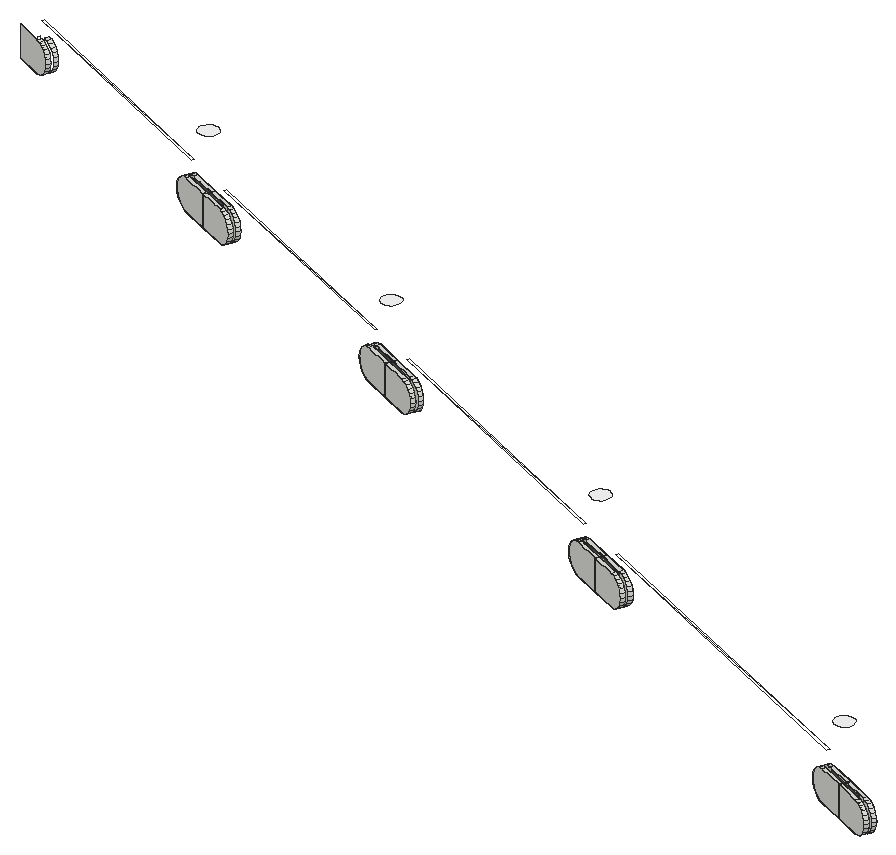
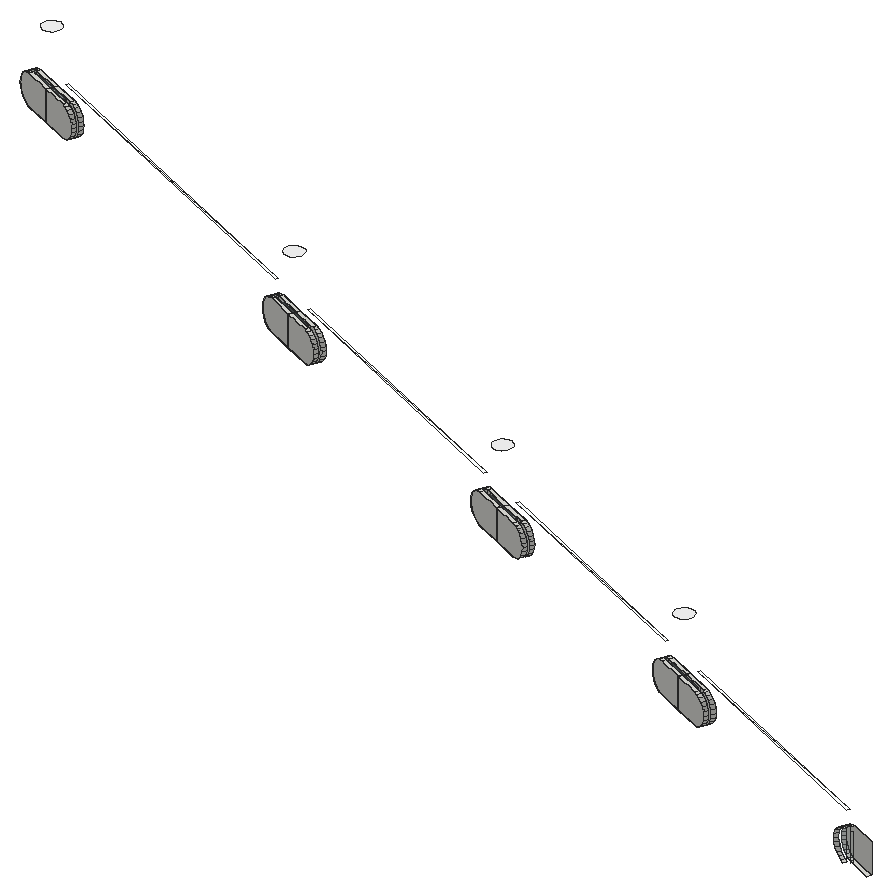
# SketchUp Ruby script. Lengths in inches.
U = 1.inch
M = Sketchup.active_model
def pt(a) = Geom::Point3d.new(a.map { |v| v * U })
def face(e, loops, mat)
  f = e.add_face(loops[0].map { |a| pt(a) })
  loops[1..].each { |l| e.add_face(l.map { |a| pt(a) }).erase! }
  f.material = f.back_material = mat if mat
  f
end
# faces: each face lists its corners as indices into pts; further lists are holes
def faces(e, pts, list, mat = nil) = list.each { |f| face(e, (f[0].is_a?(Array) ? f : [f]).map { |l| l.map { |i| pts[i] } }, mat) }
# xy, xz, yz: faces in a plane at the given z, y or x. An outline is a flat list of corners, or four numbers for a rectangle; further outlines are holes
def ring(l) = l.size == 4 ? [[l[0], l[1]], [l[2], l[1]], [l[2], l[3]], [l[0], l[3]]] : l.each_slice(2).to_a
def flat(e, list, mat, &to3) = list.each { |f| face(e, (f[0].is_a?(Array) ? f : [f]).map { |l| ring(l).map { |u, v| to3.(u, v) } }, mat) }
def xy(e, z, list, mat = nil) = flat(e, list, mat) { |x, y| [x, y, z] }
def xz(e, y, list, mat = nil) = flat(e, list, mat) { |x, z| [x, y, z] }
def yz(e, x, list, mat = nil) = flat(e, list, mat) { |y, z| [x, y, z] }
def lines(e, pts, list) = list.each { |a, b| e.add_line(pt(pts[a]), pt(pts[b])) }
# prism: a flat outline (further loops are holes) pulled along v
def prism(e, loops, v, mat = nil)
  f = face(e, loops, mat); d = Geom::Vector3d.new(v.map { |x| x * U })
  f.pushpull(f.normal.samedirection?(d) ? d.length : -d.length)
end
def box(e, o, s, mat = nil) = prism(e, [[o, [o[0] + s[0], o[1], o[2]], [o[0] + s[0], o[1] + s[1], o[2]], [o[0], o[1] + s[1], o[2]]]], [0, 0, s[2]], mat)
def at(x, y, z, deg = 0) = Geom::Transformation.translation(pt([x, y, z])) * Geom::Transformation.rotation(ORIGIN, Z_AXIS, deg.degrees)
def axes(o, x, y, z) = Geom::Transformation.new([*x, 0, *y, 0, *z, 0, *pt(o).to_a, 1])
def part(name) = M.definitions.add(name)
# library, detail: a bought-in or finely detailed component or shape, given as its bounding box
def library(name, o, s) = part(name).tap { |d| box(d.entities, o, s) }
def detail(e, o, s) = box(e.add_group.entities, o, s)
def put(e, d, t, mat = nil) = e.add_instance(d, t).tap { |i| i.material = mat if mat }
def group(e, t, mat = nil) = e.add_group.tap { |g| g.transformation = t; g.material = mat if mat }.entities
root = M.entities
M.materials.add("Glass_Safety_01").color = [204, 235, 244]
M.materials["Glass_Safety_01"].alpha = 0.1
M.materials.add("[Color_000]").color = [255, 255, 255]
xy(root,351.28,[[702.16,595.06,700.36,595.84,700.47,596.09,702.27,595.31],[702.35,595.49,700.55,596.28,700.66,596.53,702.46,595.74],[700.36,595.84,698.55,596.63,698.66,596.88,698.79,596.83,700.47,596.09],[700.55,596.28,698.87,597.01,698.74,597.0625,698.85,597.3125,700.66,596.53],[675.93,606.48,674.12,607.27,674.23,607.52,676.04,606.74],
  [676.12,606.92,674.3125,607.7,674.42,607.95,676.23,607.17],[674.12,607.27,672.32,608.05,672.43,608.31,672.57,608.24,674.23,607.52],[674.3125,607.7,672.65,608.43,672.51,608.49,672.62,608.74,674.42,607.95],[653.36,616.3125,651.55,617.1,651.66,617.35,653.47,616.57],[653.55,616.75,651.74,617.53,651.85,617.78,653.66,617],
  [651.55,617.1,649.75,617.88,649.86,618.14,650.02,618.07,651.66,617.35],[651.74,617.53,650.1,618.25,649.9375,618.32,650.05,618.57,651.85,617.78],[633.71,624.87,631.91,625.65,632.02,625.91,633.82,625.12],[633.9,625.3,632.1,626.09,632.21,626.34,634.01,625.55],[631.91,625.65,630.1,626.44,630.21,626.69,630.38,626.62,632.02,625.91],
  [632.1,626.09,630.46,626.8,630.29,626.875,630.4,627.125,632.21,626.34],[614.08,633.42,612.27,634.21,612.38,634.46,614.1875,633.67]])
xy(root,351.36,[[701.91,595.47,700.47,596.09,700.55,596.28,701.99,595.65],[700.47,596.09,699.03,596.72,699.1,596.9,700.55,596.28],[675.68,606.89,674.23,607.52,674.3125,607.7,675.76,607.07],[674.23,607.52,672.79,608.15,672.87,608.33,674.3125,607.7],[653.11,616.72,651.66,617.35,651.74,617.53,653.19,616.9],
  [651.66,617.35,650.22,617.98,650.3,618.16,651.74,617.53],[633.46,625.28,632.02,625.91,632.1,626.09,633.54,625.46],[632.02,625.91,630.57,626.54,630.65,626.72,632.1,626.09]],"Glass_Safety_01")
xy(root,353.33,[[701.91,595.47,701.99,595.65,700.55,596.28,700.47,596.09],[700.47,596.09,700.55,596.28,699.1,596.9,699.03,596.72],[675.68,606.89,675.76,607.07,674.3125,607.7,674.23,607.52],[674.23,607.52,674.3125,607.7,672.87,608.33,672.79,608.15],[653.11,616.72,653.19,616.9,651.74,617.53,651.66,617.35],
  [651.66,617.35,651.74,617.53,650.3,618.16,650.22,617.98],[633.46,625.28,633.54,625.46,632.1,626.09,632.02,625.91],[632.02,625.91,632.1,626.09,630.65,626.72,630.57,626.54]],"Glass_Safety_01")
xy(root,353.41,[[702.16,595.06,702.27,595.31,700.47,596.09,700.36,595.84],[702.35,595.49,702.46,595.74,700.66,596.53,700.55,596.28],[700.36,595.84,700.47,596.09,698.79,596.83,698.66,596.88,698.55,596.63],[700.55,596.28,700.66,596.53,698.85,597.3125,698.74,597.0625,698.87,597.01],[675.93,606.48,676.04,606.74,674.23,607.52,674.12,607.27],
  [676.12,606.92,676.23,607.17,674.42,607.95,674.3125,607.7],[674.12,607.27,674.23,607.52,672.57,608.24,672.43,608.31,672.32,608.05],[674.3125,607.7,674.42,607.95,672.62,608.74,672.51,608.49,672.65,608.43],[653.36,616.3125,653.47,616.57,651.66,617.35,651.55,617.1],[653.55,616.75,653.66,617,651.85,617.78,651.74,617.53],
  [651.55,617.1,651.66,617.35,650.02,618.07,649.86,618.14,649.75,617.88],[651.74,617.53,651.85,617.78,650.05,618.57,649.9375,618.32,650.1,618.25],[633.71,624.87,633.82,625.12,632.02,625.91,631.91,625.65],[633.9,625.3,634.01,625.55,632.21,626.34,632.1,626.09],[631.91,625.65,632.02,625.91,630.38,626.62,630.21,626.69,630.1,626.44],
  [632.1,626.09,632.21,626.34,630.4,627.125,630.29,626.875,630.46,626.8]])
xy(root,354.51,[[698.79,596.83,698.87,597.01,676.04,606.74],[698.87,597.01,676.12,606.92,676.04,606.74],[672.57,608.24,672.65,608.43,653.47,616.57],[672.65,608.43,653.55,616.75,653.47,616.57],[650.02,618.07,650.1,618.25,633.82,625.12],
  [650.1,618.25,633.9,625.3,633.82,625.12],[630.38,626.62,630.46,626.8,614.1875,633.67],[630.46,626.8,614.27,633.85,614.1875,633.67]],"Glass_Safety_01")
xy(root,357.27,[[700.55,595.56,700.71,595.59,700.86,595.66,700.98,595.77,701.08,595.91,701.13,596.07,701.14,596.23,701.1,596.39,701.03,596.54,700.92,596.66,700.78,596.75,700.63,596.8,700.46,596.8125,700.3,596.78,700.16,596.71,700.03,596.6,699.94,596.46,699.89,596.3,699.88,596.14,699.91,595.98,699.99,595.83,700.1,595.71,700.23,595.62,700.39,595.57],[674.32,606.98,674.48,607.02,674.625,607.09,674.75,607.2,674.84,607.34,674.89,607.49,674.9,607.66,674.87,607.82,674.79,607.96,674.68,608.09,674.55,608.18,674.39,608.23,674.23,608.24,674.07,608.21,673.92,608.13,673.8,608.02,673.71,607.89,673.65,607.73,673.64,607.57,673.68,607.41,673.75,607.26,673.86,607.14,674,607.05,674.15,606.99],[651.75,616.8125,651.91,616.85,652.06,616.92,652.18,617.03,652.27,617.17,652.32,617.32,652.33,617.49,652.3,617.65,652.22,617.79,652.11,617.92,651.98,618.01,651.82,618.06,651.66,618.07,651.5,618.04,651.35,617.96,651.23,617.85,651.14,617.72,651.08,617.5625,651.07,617.4,651.11,617.24,651.18,617.09,651.29,616.97,651.43,616.875,651.58,616.82],[632.1,625.37,632.26,625.4,632.41,625.48,632.53,625.59,632.625,625.72,632.68,625.88,632.69,626.04,632.65,626.2,632.58,626.35,632.47,626.47,632.33,626.5625,632.18,626.62,632.01,626.625,631.85,626.59,631.7,626.52,631.58,626.41,631.49,626.27,631.4375,626.12,631.43,625.95,631.46,625.79,631.54,625.64,631.64,625.52,631.78,625.43,631.9375,625.38]],"[Color_000]")
p = [[702.16,595.06,353.41],[700.36,595.84,353.41],[700.36,595.84,351.28],[702.16,595.06,351.28],[702.42,594.95,351.32],[702.65,594.84,351.43],
  [702.85,594.76,351.59],[703.01,594.6875,351.81],[703.11,594.65,352.07],[703.14,594.63,352.35],[703.11,594.65,352.62],[703.01,594.6875,352.88],
  [702.85,594.76,353.1],[702.65,594.84,353.27],[702.42,594.95,353.37],[702.53,595.2,351.32],[702.76,595.1,351.43],[702.27,595.31,351.28],
  [702.27,595.31,353.41],[702.96,595.01,351.59],[703.12,594.94,351.81],[703.22,594.9,352.07],[703.25,594.88,352.35],[703.22,594.9,352.62],
  [703.12,594.94,352.88],[702.96,595.01,353.1],[702.76,595.1,353.27],[702.53,595.2,353.37],[702.35,595.49,351.28],[702.35,595.49,353.41],
  [702.61,595.38,353.37],[702.84,595.28,353.27],[703.04,595.1875,353.1],[703.2,595.12,352.88],[703.29,595.08,352.62],[703.33,595.06,352.35],
  [703.29,595.08,352.07],[703.2,595.12,351.81],[703.04,595.1875,351.59],[702.84,595.28,351.43],[702.61,595.38,351.32],[700.47,596.09,353.41],
  [700.47,596.09,351.28],[700.47,596.09,351.36],[701.91,595.47,351.36],[701.91,595.47,353.33],[700.47,596.09,353.33],[700.66,596.53,353.41],
  [702.46,595.74,353.41],[702.72,595.63,353.37],[702.95,595.53,353.27],[703.15,595.44,353.1],[703.31,595.375,352.88],[703.4,595.33,352.62],
  [703.4375,595.32,352.35],[703.4,595.33,352.07],[703.31,595.375,351.81],[703.15,595.44,351.59],[702.95,595.53,351.43],[702.72,595.63,351.32],
  [702.46,595.74,351.28],[700.66,596.53,351.28],[700.55,596.28,351.28],[700.55,596.28,353.41],[700.55,596.28,353.33],[701.99,595.65,353.33],
  [701.99,595.65,351.36],[700.55,596.28,351.36],[698.55,596.63,353.41],[698.3,596.74,353.37],[698.07,596.84,353.27],[697.87,596.93,353.1],
  [697.71,597,352.88],[697.61,597.04,352.62],[697.58,597.05,352.35],[697.61,597.04,352.07],[697.71,597,351.81],[697.87,596.93,351.59],
  [698.07,596.84,351.43],[698.3,596.74,351.32],[698.55,596.63,351.28],[698.79,596.83,351.28],[698.79,596.83,353.41],[699.03,596.72,353.33],
  [699.03,596.72,351.36],[698.87,597.01,353.41],[698.87,597.01,351.28],[699.1,596.9,351.36],[699.1,596.9,353.33],[698.85,597.3125,353.41],
  [698.85,597.3125,351.28],[698.6,597.42,351.32],[698.37,597.53,351.43],[698.16,597.61,351.59],[698.01,597.68,351.81],[697.91,597.72,352.07],
  [697.88,597.74,352.35],[697.91,597.72,352.62],[698.01,597.68,352.88],[698.16,597.61,353.1],[698.37,597.53,353.27],[698.6,597.42,353.37],
  [698.41,596.99,351.32],[698.66,596.88,351.28],[698.18,597.09,351.43],[698.66,596.88,353.41],[697.98,597.18,351.59],[697.82,597.25,351.81],
  [697.72,597.29,352.07],[697.69,597.31,352.35],[697.72,597.29,352.62],[697.82,597.25,352.88],[697.98,597.18,353.1],[698.18,597.09,353.27],
  [698.41,596.99,353.37],[698.74,597.0625,351.28],[698.74,597.0625,353.41],[698.49,597.17,353.37],[698.26,597.27,353.27],[698.05,597.36,353.1],
  [697.9,597.43,352.88],[697.8,597.47,352.62],[697.77,597.49,352.35],[697.8,597.47,352.07],[697.9,597.43,351.81],[698.05,597.36,351.59],
  [698.26,597.27,351.43],[698.49,597.17,351.32],[675.93,606.48,353.41],[674.12,607.27,353.41],[674.12,607.27,351.28],[675.93,606.48,351.28],
  [676.18,606.37,351.32],[676.41,606.27,351.43],[676.62,606.18,351.59],[676.77,606.12,351.81],[676.87,606.07,352.07],[676.9,606.06,352.35],
  [676.87,606.07,352.62],[676.77,606.12,352.88],[676.62,606.18,353.1],[676.41,606.27,353.27],[676.18,606.37,353.37],[676.04,606.74,353.41],
  [676.04,606.74,351.28],[676.29,606.625,351.32],[676.52,606.52,351.43],[676.73,606.44,351.59],[676.88,606.37,351.81],[676.98,606.33,352.07],
  [677.01,606.3125,352.35],[676.98,606.33,352.62],[676.88,606.37,352.88],[676.73,606.44,353.1],[676.52,606.52,353.27],[676.29,606.625,353.37],
  [676.12,606.92,351.28],[676.12,606.92,353.41],[676.37,606.81,353.37],[676.6,606.7,353.27],[676.81,606.62,353.1],[676.96,606.55,352.88],
  [677.06,606.51,352.62],[677.09,606.49,352.35],[677.06,606.51,352.07],[676.96,606.55,351.81],[676.81,606.62,351.59],[676.6,606.7,351.43],
  [676.37,606.81,351.32],[674.23,607.52,353.41],[674.23,607.52,351.28],[674.23,607.52,351.36],[675.68,606.89,351.36],[675.68,606.89,353.33],
  [674.23,607.52,353.33],[674.42,607.95,353.41],[676.23,607.17,353.41],[676.48,607.06,353.37],[676.71,606.96,353.27],[676.92,606.87,353.1],
  [677.07,606.8,352.88],[677.17,606.76,352.62],[677.2,606.74,352.35],[677.17,606.76,352.07],[677.07,606.8,351.81],[676.92,606.87,351.59],
  [676.71,606.96,351.43],[676.48,607.06,351.32],[676.23,607.17,351.28],[674.42,607.95,351.28],[674.3125,607.7,351.28],[674.3125,607.7,353.41],
  [674.3125,607.7,353.33],[675.76,607.07,353.33],[675.76,607.07,351.36],[674.3125,607.7,351.36],[672.32,608.05,353.41],[672.07,608.16,353.37],
  [671.83,608.27,353.27],[671.63,608.36,353.1],[671.47,608.42,352.88],[671.375,608.46,352.62],[671.34,608.48,352.35],[671.375,608.46,352.07],
  [671.47,608.42,351.81],[671.63,608.36,351.59],[671.83,608.27,351.43],[672.07,608.16,351.32],[672.32,608.05,351.28],[672.57,608.24,351.28],
  [672.57,608.24,353.41],[672.79,608.15,353.33],[672.79,608.15,351.36],[672.65,608.43,353.41],[672.65,608.43,351.28],[672.87,608.33,351.36],
  [672.87,608.33,353.33],[672.62,608.74,353.41],[672.62,608.74,351.28],[672.36,608.85,351.32],[672.13,608.95,351.43],[671.93,609.04,351.59],
  [671.77,609.11,351.81],[671.68,609.15,352.07],[671.64,609.17,352.35],[671.68,609.15,352.62],[671.77,609.11,352.88],[671.93,609.04,353.1],
  [672.13,608.95,353.27],[672.36,608.85,353.37],[672.18,608.42,351.32],[672.43,608.31,351.28],[672.43,608.31,353.41],[671.94,608.52,351.43],
  [671.74,608.61,351.59],[671.58,608.68,351.81],[671.49,608.72,352.07],[671.45,608.73,352.35],[671.49,608.72,352.62],[671.58,608.68,352.88],
  [671.74,608.61,353.1],[671.94,608.52,353.27],[672.18,608.42,353.37],[672.51,608.49,351.28],[672.51,608.49,353.41],[672.25,608.6,353.37],
  [672.02,608.7,353.27],[671.82,608.79,353.1],[671.66,608.86,352.88],[671.57,608.9,352.62],[671.53,608.91,352.35],[671.57,608.9,352.07],
  [671.66,608.86,351.81],[671.82,608.79,351.59],[672.02,608.7,351.43],[672.25,608.6,351.32],[653.36,616.3125,353.41],[651.55,617.1,353.41],
  [651.55,617.1,351.28],[653.36,616.3125,351.28],[653.61,616.2,351.32],[653.84,616.1,351.43],[654.05,616.01,351.59],[654.2,615.95,351.81],
  [654.3,615.9,352.07],[654.33,615.89,352.35],[654.3,615.9,352.62],[654.2,615.95,352.88],[654.05,616.01,353.1],[653.84,616.1,353.27],
  [653.61,616.2,353.37],[653.47,616.57,353.41],[653.47,616.57,351.28],[653.72,616.46,351.32],[653.96,616.35,351.43],[654.16,616.27,351.59],
  [654.3125,616.2,351.81],[654.41,616.16,352.07],[654.44,616.14,352.35],[654.41,616.16,352.62],[654.3125,616.2,352.88],[654.16,616.27,353.1],
  [653.96,616.35,353.27],[653.72,616.46,353.37],[653.55,616.75,351.28],[653.55,616.75,353.41],[653.8,616.64,353.37],[654.03,616.53,353.27],
  [654.24,616.45,353.1],[654.39,616.38,352.88],[654.49,616.34,352.62],[654.52,616.32,352.35],[654.49,616.34,352.07],[654.39,616.38,351.81],
  [654.24,616.45,351.59],[654.03,616.53,351.43],[653.8,616.64,351.32],[653.91,616.89,351.32],[654.14,616.79,351.43],[651.66,617.35,353.41],
  [651.66,617.35,351.28],[651.66,617.35,351.36],[653.11,616.72,351.36],[653.11,616.72,353.33],[651.66,617.35,353.33],[651.85,617.78,353.41],
  [653.66,617,353.41],[653.91,616.89,353.37],[654.14,616.79,353.27],[654.35,616.7,353.1],[654.5,616.63,352.88],[654.6,616.59,352.62],
  [654.63,616.57,352.35],[654.6,616.59,352.07],[654.5,616.63,351.81],[654.35,616.7,351.59],[653.66,617,351.28],[651.85,617.78,351.28],
  [651.74,617.53,351.28],[651.74,617.53,353.41],[651.74,617.53,353.33],[653.19,616.9,353.33],[653.19,616.9,351.36],[651.74,617.53,351.36],
  [649.75,617.88,353.41],[649.5,617.99,353.37],[649.26,618.1,353.27],[649.06,618.18,353.1],[648.9,618.25,352.88],[648.81,618.29,352.62],
  [648.77,618.31,352.35],[648.81,618.29,352.07],[648.9,618.25,351.81],[649.06,618.18,351.59],[649.26,618.1,351.43],[649.5,617.99,351.32],
  [649.75,617.88,351.28],[650.02,618.07,351.28],[650.02,618.07,353.41],[650.22,617.98,353.33],[650.22,617.98,351.36],[650.1,618.25,353.41],
  [650.1,618.25,351.28],[650.3,618.16,351.36],[650.3,618.16,353.33],[650.05,618.57,353.41],[650.05,618.57,351.28],[649.79,618.68,351.32],
  [649.56,618.78,351.43],[649.36,618.87,351.59],[649.2,618.9375,351.81],[649.11,618.98,352.07],[649.07,618.99,352.35],[649.11,618.98,352.62],
  [649.2,618.9375,352.88],[649.36,618.87,353.1],[649.56,618.78,353.27],[649.79,618.68,353.37],[649.61,618.25,351.32],[649.86,618.14,351.28],
  [649.37,618.35,351.43],[649.86,618.14,353.41],[649.17,618.4375,351.59],[649.01,618.5,351.81],[648.92,618.55,352.07],[648.88,618.5625,352.35],
  [648.92,618.55,352.62],[649.01,618.5,352.88],[649.17,618.4375,353.1],[649.37,618.35,353.27],[649.61,618.25,353.37],[649.9375,618.32,351.28],
  [649.9375,618.32,353.41],[649.68,618.43,353.37],[649.45,618.53,353.27],[649.25,618.62,353.1],[649.09,618.69,352.88],[649,618.73,352.62],
  [648.96,618.74,352.35],[649,618.73,352.07],[649.09,618.69,351.81],[649.25,618.62,351.59],[649.45,618.53,351.43],[649.68,618.43,351.32],
  [633.71,624.87,353.41],[631.91,625.65,353.41],[631.91,625.65,351.28],[633.71,624.87,351.28],[633.96,624.76,351.32],[634.2,624.66,351.43],
  [634.4,624.57,351.59],[634.56,624.5,351.81],[634.65,624.46,352.07],[634.6875,624.44,352.35],[634.65,624.46,352.62],[634.56,624.5,352.88],
  [634.4,624.57,353.1],[634.2,624.66,353.27],[633.96,624.76,353.37],[633.82,625.12,353.41],[633.82,625.12,351.28],[634.07,625.01,351.32],
  [634.31,624.91,351.43],[634.51,624.82,351.59],[634.67,624.75,351.81],[634.76,624.71,352.07],[634.8,624.7,352.35],[634.76,624.71,352.62],
  [634.67,624.75,352.88],[634.51,624.82,353.1],[634.31,624.91,353.27],[634.07,625.01,353.37],[633.9,625.3,351.28],[633.9,625.3,353.41],
  [634.15,625.19,353.37],[634.39,625.09,353.27],[634.59,625,353.1],[634.75,624.93,352.88],[634.84,624.89,352.62],[634.875,624.88,352.35],
  [634.84,624.89,352.07],[634.75,624.93,351.81],[634.59,625,351.59],[634.39,625.09,351.43],[634.15,625.19,351.32],[632.02,625.91,353.41],
  [632.02,625.91,351.28],[632.02,625.91,351.36],[633.46,625.28,351.36],[633.46,625.28,353.33],[632.02,625.91,353.33],[632.21,626.34,353.41],
  [634.01,625.55,353.41],[634.26,625.44,353.37],[634.5,625.34,353.27],[634.7,625.25,353.1],[634.86,625.1875,352.88],[634.95,625.14,352.62],
  [634.99,625.13,352.35],[634.95,625.14,352.07],[634.86,625.1875,351.81],[634.7,625.25,351.59],[634.5,625.34,351.43],[634.26,625.44,351.32],
  [634.01,625.55,351.28],[632.21,626.34,351.28],[632.1,626.09,351.28],[632.1,626.09,353.41],[632.1,626.09,353.33],[633.54,625.46,353.33],
  [633.54,625.46,351.36],[632.1,626.09,351.36],[630.1,626.44,353.41],[629.85,626.55,353.37],[629.62,626.65,353.27],[629.41,626.74,353.1],
  [629.26,626.81,352.88],[629.16,626.85,352.62],[629.13,626.87,352.35],[629.16,626.85,352.07],[629.26,626.81,351.81],[629.41,626.74,351.59],
  [629.62,626.65,351.43],[629.85,626.55,351.32],[630.1,626.44,351.28],[630.38,626.62,351.28],[630.38,626.62,353.41],[630.57,626.54,353.33],
  [630.57,626.54,351.36],[630.46,626.8,353.41],[630.46,626.8,351.28],[630.65,626.72,351.36],[630.65,626.72,353.33],[630.4,627.125,353.41],
  [630.4,627.125,351.28],[630.15,627.24,351.32],[629.91,627.34,351.43],[629.71,627.43,351.59],[629.56,627.49,351.81],[629.46,627.54,352.07],
  [629.43,627.55,352.35],[629.46,627.54,352.62],[629.56,627.49,352.88],[629.71,627.43,353.1],[629.91,627.34,353.27],[630.15,627.24,353.37],
  [629.96,626.8,351.32],[630.21,626.69,351.28],[630.21,626.69,353.41],[629.73,626.91,351.43],[629.52,626.99,351.59],[629.37,627.0625,351.81],
  [629.27,627.1,352.07],[629.24,627.12,352.35],[629.27,627.1,352.62],[629.37,627.0625,352.88],[629.52,626.99,353.1],[629.73,626.91,353.27],
  [629.96,626.8,353.37],[630.29,626.875,351.28],[630.29,626.875,353.41],[630.04,626.98,353.37],[629.8,627.09,353.27],[629.6,627.17,353.1],
  [629.45,627.24,352.88],[629.35,627.28,352.62],[629.32,627.3,352.35],[629.35,627.28,352.07],[629.45,627.24,351.81],[629.6,627.17,351.59],
  [629.8,627.09,351.43],[630.04,626.98,351.32],[614.08,633.42,353.41],[612.27,634.21,353.41],[612.27,634.21,351.28],[614.08,633.42,351.28],
  [614.33,633.3125,351.32],[614.5625,633.21,351.43],[614.77,633.12,351.59],[614.92,633.05,351.81],[615.02,633.01,352.07],[615.05,633,352.35],
  [615.02,633.01,352.62],[614.92,633.05,352.88],[614.77,633.12,353.1],[614.5625,633.21,353.27],[614.33,633.3125,353.37],[614.1875,633.67,353.41],
  [614.1875,633.67,351.28],[614.4375,633.5625,351.32],[614.67,633.46,351.43],[614.875,633.375,351.59],[615.03,633.31,351.81],[615.13,633.26,352.07],
  [615.16,633.25,352.35],[615.13,633.26,352.62],[615.03,633.31,352.88],[614.875,633.375,353.1],[614.67,633.46,353.27],[614.4375,633.5625,353.37],
  [614.27,633.85,351.28],[614.27,633.85,353.41],[614.52,633.74,353.37],[614.75,633.64,353.27],[614.95,633.55,353.1],[615.11,633.49,352.88],
  [615.21,633.44,352.62],[615.24,633.43,352.35],[615.21,633.44,352.07],[615.11,633.49,351.81],[614.95,633.55,351.59],[614.75,633.64,351.43],
  [614.52,633.74,351.32],[614.63,634,351.32],[614.86,633.89,351.43],[614.375,634.11,351.28],[615.06,633.81,351.59],[613.83,633.83,353.33],
  [613.83,633.83,351.36],[613.9,634.01,351.36],[613.9,634.01,353.33],[615.22,633.74,351.81],[615.32,633.7,352.07],[615.35,633.68,352.35],
  [615.32,633.7,352.62],[615.22,633.74,352.88],[615.06,633.81,353.1],[614.86,633.89,353.27],[614.63,634,353.37],[614.375,634.11,353.41]]
faces(root,p,[[0,1,2,3,4,5,6,7,8,9,10,11,12,13,14],[15,16,5,4],[17,15,4,3],[41,18,17,42,43,44,45,46],[47,48,49,50,51,52,53,54,55,56,57,58,59,60,61],[39,40,59,58],[40,28,60,59],[62,28,29,63,64,65,66,67],
  [1,68,69,70,71,72,73,74,75,76,77,78,79,80,2],[42,43,46,41,1,2],[42,81,82,41,46,83,84,43],[63,85,86,62,67,87,88,64],[67,62,61,47,63,64],[89,47,61,90,91,92,93,94,95,96,97,98,99,100,101],[102,103,80,79],[104,102,79,78],
  [105,82,81,103,102,104,106,107,108,109,110,111,112,113,114],[115,86,85,116,117,118,119,120,121,122,123,124,125,126,127],[115,127,91,90],[127,126,92,91],[128,129,130,131,132,133,134,135,136,137,138,139,140,141,142],[145,146,133,132],[144,145,132,131],[169,143,144,170,171,172,173,174],
  [175,176,177,178,179,180,181,182,183,184,185,186,187,188,189],[167,168,187,186],[168,156,188,187],[190,156,157,191,192,193,194,195],[129,196,197,198,199,200,201,202,203,204,205,206,207,208,130],[170,171,174,169,129,130],[170,209,210,169,174,211,212,171],[191,213,214,190,195,215,216,192],
  [195,190,189,175,191,192],[217,175,189,218,219,220,221,222,223,224,225,226,227,228,229],[230,231,208,207],[232,210,209,231,230,233,234,235,236,237,238,239,240,241,242],[233,230,207,206],[243,214,213,244,245,246,247,248,249,250,251,252,253,254,255],[243,255,219,218],[255,254,220,219],
  [256,257,258,259,260,261,262,263,264,265,266,267,268,269,270],[273,274,261,260],[272,273,260,259],[295,296,297,298],[299,271,272,300,301,302,303,304],[305,306,307,308,309,310,311,312,313,314,315,298,297,316,317],[296,284,316,297],[318,284,285,319,320,321,322,323],
  [257,324,325,326,327,328,329,330,331,332,333,334,335,336,258],[300,301,304,299,257,258],[300,337,338,299,304,339,340,301],[319,341,342,318,323,343,344,320],[323,318,317,305,319,320],[345,305,317,346,347,348,349,350,351,352,353,354,355,356,357],[358,359,336,335],[360,358,335,334],
  [361,338,337,359,358,360,362,363,364,365,366,367,368,369,370],[371,342,341,372,373,374,375,376,377,378,379,380,381,382,383],[371,383,347,346],[383,382,348,347],[384,385,386,387,388,389,390,391,392,393,394,395,396,397,398],[401,402,389,388],[400,401,388,387],[425,399,400,426,427,428,429,430],
  [431,432,433,434,435,436,437,438,439,440,441,442,443,444,445],[423,424,443,442],[424,412,444,443],[446,412,413,447,448,449,450,451],[385,452,453,454,455,456,457,458,459,460,461,462,463,464,386],[426,427,430,425,385,386],[426,465,466,425,430,467,468,427],[447,469,470,446,451,471,472,448],
  [451,446,445,431,447,448],[473,431,445,474,475,476,477,478,479,480,481,482,483,484,485],[486,487,464,463],[488,466,465,487,486,489,490,491,492,493,494,495,496,497,498],[489,486,463,462],[499,470,469,500,501,502,503,504,505,506,507,508,509,510,511],[499,511,475,474],[511,510,476,475],
  [512,513,514,515,516,517,518,519,520,521,522,523,524,525,526],[529,530,517,516],[528,529,516,515],[551,552,553,554],[552,540,555,553],[16,19,6,5],[38,39,58,57],[106,104,78,77],
  [126,125,93,92],[146,147,134,133],[166,167,186,185],[234,233,206,205],[254,253,221,220],[274,275,262,261],[294,295,298,315],[362,360,334,333],
  [382,381,349,348],[402,403,390,389],[422,423,442,441],[490,489,462,461],[510,509,477,476],[530,531,518,517],[550,551,554,556],[19,20,7,6],
  [37,38,57,56],[107,106,77,76],[125,124,94,93],[147,148,135,134],[165,166,185,184],[235,234,205,204],[253,252,222,221],[275,276,263,262],
  [293,294,315,314],[363,362,333,332],[381,380,350,349],[403,404,391,390],[421,422,441,440],[491,490,461,460],[509,508,478,477],[531,532,519,518],
  [549,550,556,561],[20,21,8,7],[36,37,56,55],[108,107,76,75],[124,123,95,94],[148,149,136,135],[164,165,184,183],[236,235,204,203],
  [252,251,223,222],[276,277,264,263],[292,293,314,313],[364,363,332,331],[380,379,351,350],[404,405,392,391],[420,421,440,439],[492,491,460,459],
  [508,507,479,478],[532,533,520,519],[548,549,561,562],[21,22,9,8],[35,36,55,54],[109,108,75,74],[123,122,96,95],[149,150,137,136],
  [163,164,183,182],[237,236,203,202],[251,250,224,223],[277,278,265,264],[291,292,313,312],[365,364,331,330],[379,378,352,351],[405,406,393,392],
  [419,420,439,438],[493,492,459,458],[507,506,480,479],[533,534,521,520],[547,548,562,563],[22,23,10,9],[34,35,54,53],[110,109,74,73],
  [122,121,97,96],[150,151,138,137],[162,163,182,181],[238,237,202,201],[250,249,225,224],[278,279,266,265],[290,291,312,311],[366,365,330,329],
  [378,377,353,352],[406,407,394,393],[418,419,438,437],[494,493,458,457],[506,505,481,480],[534,535,522,521],[546,547,563,564],[23,24,11,10],
  [33,34,53,52],[111,110,73,72],[121,120,98,97],[151,152,139,138],[161,162,181,180],[239,238,201,200],[249,248,226,225],[279,280,267,266],
  [289,290,311,310],[367,366,329,328],[377,376,354,353],[407,408,395,394],[417,418,437,436],[495,494,457,456],[505,504,482,481],[535,536,523,522],
  [545,546,564,565],[24,25,12,11],[32,33,52,51],[112,111,72,71],[120,119,99,98],[152,153,140,139],[160,161,180,179],[240,239,200,199],
  [248,247,227,226],[280,281,268,267],[288,289,310,309],[368,367,328,327],[376,375,355,354],[408,409,396,395],[416,417,436,435],[496,495,456,455],
  [504,503,483,482],[536,537,524,523],[544,545,565,566],[25,26,13,12],[31,32,51,50],[113,112,71,70],[119,118,100,99],[153,154,141,140],
  [159,160,179,178],[241,240,199,198],[247,246,228,227],[281,282,269,268],[287,288,309,308],[369,368,327,326],[375,374,356,355],[409,410,397,396],
  [415,416,435,434],[497,496,455,454],[503,502,484,483],[537,538,525,524],[543,544,566,567],[26,27,14,13],[30,31,50,49],[114,113,70,69],
  [118,117,101,100],[154,155,142,141],[158,159,178,177],[242,241,198,197],[246,245,229,228],[282,283,270,269],[286,287,308,307],[370,369,326,325],
  [374,373,357,356],[410,411,398,397],[414,415,434,433],[498,497,454,453],[502,501,485,484],[538,539,526,525],[542,543,567,568],[27,18,0,14],
  [29,30,49,48],[105,114,69,68],[117,116,89,101],[155,143,128,142],[157,158,177,176],[232,242,197,196],[245,244,217,229],[283,271,256,270],
  [285,286,307,306],[361,370,325,324],[373,372,345,357],[411,399,384,398],[413,414,433,432],[488,498,453,452],[501,500,473,485],[539,527,512,526],
  [541,542,568,569]])
faces(root,p,[[18,17,15,16,19,20,21,22,23,24,25,26,27],[28,29,30,31,32,33,34,35,36,37,38,39,40],[143,144,145,146,147,148,149,150,151,152,153,154,155],[156,157,158,159,160,161,162,163,164,165,166,167,168],[271,272,273,274,275,276,277,278,279,280,281,282,283],[284,285,286,287,288,289,290,291,292,293,294,295,296],[399,400,401,402,403,404,405,406,407,408,409,410,411],[412,413,414,415,416,417,418,419,420,421,422,423,424],
  [527,528,529,530,531,532,533,534,535,536,537,538,539],[540,541,542,543,544,545,546,547,548,549,550,551,552],[46,45,44,43],[45,44,66,65],[65,64,67,66],[83,46,43,84],[64,46,43,67],[64,88,87,67],
  [88,87,84,83],[174,173,172,171],[173,172,194,193],[193,192,195,194],[211,174,171,212],[192,174,171,195],[192,216,215,195],[216,215,212,211],
  [304,303,302,301],[303,302,322,321],[321,320,323,322],[339,304,301,340],[320,304,301,323],[320,344,343,323],[344,343,340,339],[430,429,428,427],
  [429,428,450,449],[449,448,451,450],[467,430,427,468],[448,430,427,451],[448,472,471,451],[472,471,468,467],[557,558,559,560]],"Glass_Safety_01")
